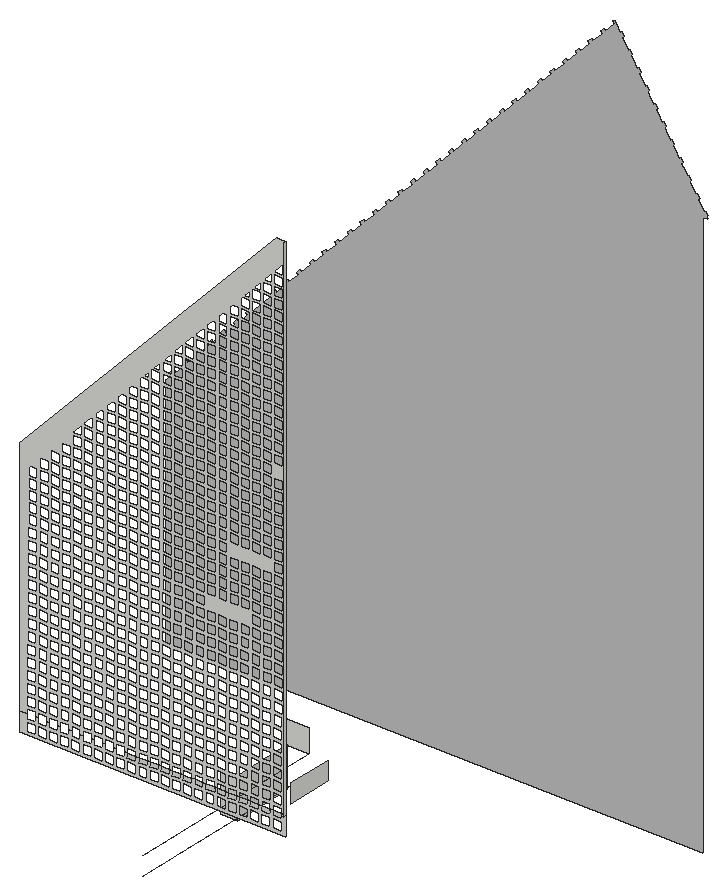
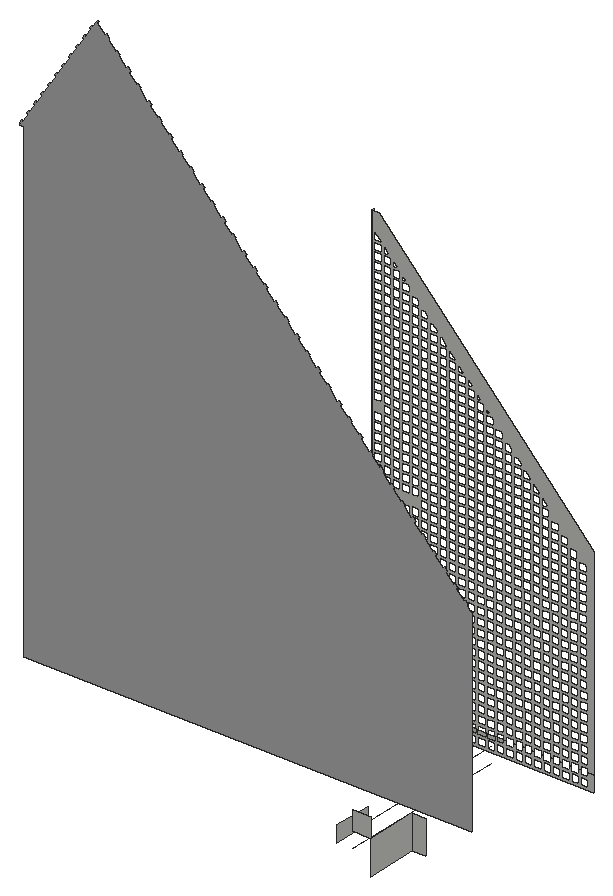
# SketchUp Ruby script. Lengths in inches.
U = 1.inch
M = Sketchup.active_model
def pt(a) = Geom::Point3d.new(a.map { |v| v * U })
def face(e, loops, mat)
  f = e.add_face(loops[0].map { |a| pt(a) })
  loops[1..].each { |l| e.add_face(l.map { |a| pt(a) }).erase! }
  f.material = f.back_material = mat if mat
  f
end
# faces: each face lists its corners as indices into pts; further lists are holes
def faces(e, pts, list, mat = nil) = list.each { |f| face(e, (f[0].is_a?(Array) ? f : [f]).map { |l| l.map { |i| pts[i] } }, mat) }
# xy, xz, yz: faces in a plane at the given z, y or x. An outline is a flat list of corners, or four numbers for a rectangle; further outlines are holes
def ring(l) = l.size == 4 ? [[l[0], l[1]], [l[2], l[1]], [l[2], l[3]], [l[0], l[3]]] : l.each_slice(2).to_a
def flat(e, list, mat, &to3) = list.each { |f| face(e, (f[0].is_a?(Array) ? f : [f]).map { |l| ring(l).map { |u, v| to3.(u, v) } }, mat) }
def xy(e, z, list, mat = nil) = flat(e, list, mat) { |x, y| [x, y, z] }
def xz(e, y, list, mat = nil) = flat(e, list, mat) { |x, z| [x, y, z] }
def yz(e, x, list, mat = nil) = flat(e, list, mat) { |y, z| [x, y, z] }
def lines(e, pts, list) = list.each { |a, b| e.add_line(pt(pts[a]), pt(pts[b])) }
# prism: a flat outline (further loops are holes) pulled along v
def prism(e, loops, v, mat = nil)
  f = face(e, loops, mat); d = Geom::Vector3d.new(v.map { |x| x * U })
  f.pushpull(f.normal.samedirection?(d) ? d.length : -d.length)
end
def box(e, o, s, mat = nil) = prism(e, [[o, [o[0] + s[0], o[1], o[2]], [o[0] + s[0], o[1] + s[1], o[2]], [o[0], o[1] + s[1], o[2]]]], [0, 0, s[2]], mat)
def at(x, y, z, deg = 0) = Geom::Transformation.translation(pt([x, y, z])) * Geom::Transformation.rotation(ORIGIN, Z_AXIS, deg.degrees)
def axes(o, x, y, z) = Geom::Transformation.new([*x, 0, *y, 0, *z, 0, *pt(o).to_a, 1])
def part(name) = M.definitions.add(name)
# library, detail: a bought-in or finely detailed component or shape, given as its bounding box
def library(name, o, s) = part(name).tap { |d| box(d.entities, o, s) }
def detail(e, o, s) = box(e.add_group.entities, o, s)
def put(e, d, t, mat = nil) = e.add_instance(d, t).tap { |i| i.material = mat if mat }
def group(e, t, mat = nil) = e.add_group.tap { |g| g.transformation = t; g.material = mat if mat }.entities
root = M.entities
M.materials.add("[Color M02]").color = [198, 198, 198]
xz(root,480.77,[[[2203.9,258.95,2203.9,263.89,2205.69,263.89,2205.69,262.73,2208,262.73,2208,263.89,2208.6,263.89,2208.6,262.73,2210.92,262.73,2210.92,263.89,2211.52,263.89,2211.52,262.73,2213.83,262.73,2213.83,263.89,2214.43,263.89,2214.43,262.73,2216.74,262.73,2216.74,263.89,2217.34,263.89,2217.34,262.73,2219.65,262.73,2219.65,263.89,2220.25,263.89,2220.25,262.73,2222.5625,262.73,2222.5625,263.89,2223.16,263.89,2223.16,262.73,2225.48,262.73,2225.48,263.89,2226.08,263.89,2226.08,262.73,2228.39,262.73,2228.39,263.89,2228.99,263.89,2228.99,262.73,2231.3,262.73,2231.3,263.89,2231.9,263.89,2231.9,262.73,2234.21,262.73,2234.21,263.89,2234.8125,263.89,2234.8125,262.73,2237.125,262.73,2237.125,263.89,2237.72,263.89,2237.72,262.73,2240.04,262.73,2240.04,263.89,2240.64,263.89,2240.64,262.73,2242.95,262.73,2242.95,263.89,2243.55,263.89,2243.55,262.73,2245.86,262.73,2245.86,263.89,2246.46,263.89,2246.46,262.73,2248.77,262.73,2248.77,263.89,2249.37,263.89,2249.37,262.73,2251.68,262.73,2251.68,263.89,2252.28,263.89,2252.28,262.73,2254.6,262.73,2254.6,263.89,2255.2,263.89,2255.2,262.73,2257.51,262.73,2257.51,263.89,2258.11,263.89,2258.11,262.73,2260.42,262.73,2260.42,263.89,2261.02,263.89,2261.02,262.73,2263.33,262.73,2263.33,263.89,2263.93,263.89,2263.93,262.73,2266.24,262.73,2266.24,263.89,2266.84,263.89,2266.84,262.73,2269.16,262.73,2269.16,263.89,2269.76,263.89,2269.76,262.73,2272.07,262.73,2272.07,263.89,2273.22,263.89,2273.22,258.95],[2269.73,259.68,2272.04,262],[2266.81,259.68,2269.13,262],[2263.9,259.68,2266.22,262],[2260.99,259.68,2263.3,262],[2258.08,259.68,2260.39,262],[2255.17,259.68,2257.48,262],[2252.25,259.68,2254.57,262],[2249.34,259.68,2251.66,262],[2246.43,259.68,2248.74,262],[2243.52,259.68,2245.83,262],[2240.61,259.68,2242.92,262],[2237.69,259.68,2240.01,262],[2234.78,259.68,2237.09,262],[2231.87,259.68,2234.18,262],[2228.96,259.68,2231.27,262],[2226.05,259.68,2228.36,262],[2223.13,259.68,2225.45,262],[2220.22,259.68,2222.53,262],[2217.31,259.68,2219.62,262],[2214.4,259.68,2216.71,262],[2211.49,259.68,2213.8,262],[2208.57,259.68,2210.89,262],[2205.66,259.68,2207.97,262]],[2231.9,262.73,2234.21,263.89],[2234.8125,262.73,2237.125,263.89],[2237.72,262.73,2240.04,263.89],[2240.64,262.73,2242.95,263.89],
  [2243.55,262.73,2245.86,263.89],[2246.46,262.73,2248.77,263.89],[2249.37,262.73,2251.68,263.89],[2252.28,262.73,2254.6,263.89],[2255.2,262.73,2257.51,263.89],
  [2258.11,262.73,2260.42,263.89],[2261.02,262.73,2263.33,263.89],[2263.93,262.73,2266.24,263.89],[2266.84,262.73,2269.16,263.89],[2269.76,262.73,2272.07,263.89],
  [[2203.9,263.89,2203.9,326.5,2270.96,397.75,2273.22,397.75,2273.22,263.89,2272.07,263.89,2272.07,265.04,2269.76,265.04,2269.76,263.89,2269.16,263.89,2269.16,265.04,2266.84,265.04,2266.84,263.89,2266.24,263.89,2266.24,265.04,2263.93,265.04,2263.93,263.89,2263.33,263.89,2263.33,265.04,2261.02,265.04,2261.02,263.89,2260.42,263.89,2260.42,265.04,2258.11,265.04,2258.11,263.89,2257.51,263.89,2257.51,265.04,2255.2,265.04,2255.2,263.89,2254.6,263.89,2254.6,265.04,2252.28,265.04,2252.28,263.89,2251.68,263.89,2251.68,265.04,2249.37,265.04,2249.37,263.89,2248.77,263.89,2248.77,265.04,2246.46,265.04,2246.46,263.89,2245.86,263.89,2245.86,265.04,2243.55,265.04,2243.55,263.89,2242.95,263.89,2242.95,265.04,2240.64,265.04,2240.64,263.89,2240.04,263.89,2240.04,265.04,2237.72,265.04,2237.72,263.89,2237.125,263.89,2237.125,265.04,2234.8125,265.04,2234.8125,263.89,2234.21,263.89,2234.21,265.04,2231.9,265.04,2231.9,263.89,2231.3,263.89,2231.3,265.04,2228.99,265.04,2228.99,263.89,2228.39,263.89,2228.39,265.04,2226.08,265.04,2226.08,263.89,2225.48,263.89,2225.48,265.04,2223.16,265.04,2223.16,263.89,2222.5625,263.89,2222.5625,265.04,2220.25,265.04,2220.25,263.89,2219.65,263.89,2219.65,265.04,2217.34,265.04,2217.34,263.89,2216.74,263.89,2216.74,265.04,2214.43,265.04,2214.43,263.89,2213.83,263.89,2213.83,265.04,2211.52,265.04,2211.52,263.89,2210.92,263.89,2210.92,265.04,2208.6,265.04,2208.6,263.89,2208,263.89,2208,265.04,2205.69,265.04,2205.69,263.89],[2258.52,370.27,2260.86,372.59],[2270.19,386.84,2272.5,389.15],[2270.19,384.09,2272.5,386.4],[2267.28,384.09,2269.59,386.4],[2267.25,381.34,2269.57,383.65],[2270.19,381.34,2272.5,383.65],[2270.19,378.59,2272.5,380.9],[2267.25,378.59,2269.57,380.9],[2264.34,375.84,2266.65,378.15],[2267.28,375.84,2269.59,378.15],[2270.19,375.84,2272.5,378.15],[2270.19,373.09,2272.5,375.4],[2267.25,373.09,2269.57,375.4],[2264.37,373.09,2266.68,375.4],[2261.43,373.09,2263.74,375.4],[2267.25,370.27,2269.57,372.59],[2270.19,370.27,2272.5,372.59],[2261.45,370.27,2263.77,372.59],[2255.63,370.27,2257.94,372.59],[2252.72,367.46,2255.03,369.77],[2255.63,367.46,2257.94,369.77],[2258.54,367.46,2260.86,369.77],[2261.45,367.46,2263.77,369.77],[2264.37,367.46,2266.68,369.77],[2267.28,367.46,2269.59,369.77],[2270.19,367.46,2272.5,369.77],[2270.19,364.65,2272.5,366.96],[2267.28,364.65,2269.59,366.96],[2264.37,364.65,2266.68,366.96],[2261.45,364.65,2263.77,366.96],[2258.54,364.65,2260.86,366.96],[2255.63,364.65,2257.94,366.96],[2252.72,364.65,2255.03,366.96],[2249.81,364.65,2252.12,366.96],[2246.89,361.84,2249.21,364.15],[2249.81,361.84,2252.12,364.15],[2252.72,361.84,2255.03,364.15],[2255.63,361.84,2257.94,364.15],[2258.54,361.84,2260.86,364.15],[2261.45,361.84,2263.77,364.15],[2264.37,361.84,2266.68,364.15],[2267.28,361.84,2269.59,364.15],[2270.19,361.84,2272.5,364.15],[2270.19,359.02,2272.5,361.34],[2267.28,359.02,2269.59,361.34],[2264.37,359.02,2266.68,361.34],[2261.45,359.02,2263.77,361.34],[2258.54,359.02,2260.86,361.34],[2255.63,359.02,2257.94,361.34],[2252.72,359.02,2255.03,361.34],[2249.81,359.02,2252.12,361.34],[2246.89,359.02,2249.21,361.34],[2243.98,359.02,2246.29,361.34],[2241.07,356.21,2243.38,358.52],[2243.98,356.21,2246.29,358.52],[2246.89,356.21,2249.21,358.52],[2249.81,356.21,2252.12,358.52],[2252.72,356.21,2255.03,358.52],[2255.63,356.21,2257.94,358.52],[2258.54,356.21,2260.86,358.52],[2261.45,356.21,2263.77,358.52],[2264.37,356.21,2266.68,358.52],[2267.28,356.21,2269.59,358.52],[2270.19,356.21,2272.5,358.52],[2238.16,350.59,2240.47,352.9],[2241.07,353.4,2243.38,355.71],[2241.07,350.59,2243.38,352.9],[2243.98,350.59,2246.29,352.9],[2243.98,353.4,2246.29,355.71],[2246.89,353.4,2249.21,355.71],[2246.89,350.59,2249.21,352.9],[2249.81,353.4,2252.12,355.71],[2249.81,350.59,2252.12,352.9],[2252.72,353.4,2255.03,355.71],[2252.72,350.59,2255.03,352.9],[2255.63,353.4,2257.94,355.71],[2255.63,350.59,2257.94,352.9],[2258.54,353.4,2260.86,355.71],[2258.54,350.59,2260.86,352.9],[2261.45,350.59,2263.77,352.9],[2261.45,353.4,2263.77,355.71],[2264.37,353.4,2266.68,355.71],[2267.28,353.4,2269.59,355.71],[2270.19,353.4,2272.5,355.71],[2270.19,350.59,2272.5,352.9],[2267.28,350.59,2269.59,352.9],[2264.37,350.59,2266.68,352.9],[2270.19,347.77,2272.5,350.09],[2267.28,347.77,2269.59,350.09],[2264.37,347.77,2266.68,350.09],[2261.45,347.77,2263.77,350.09],[2258.54,347.77,2260.86,350.09],[2255.63,347.77,2257.94,350.09],[2252.72,347.77,2255.03,350.09],[2249.81,347.77,2252.12,350.09],[2246.89,347.77,2249.21,350.09],[2243.98,347.77,2246.29,350.09],[2241.07,347.77,2243.38,350.09],[2238.16,347.77,2240.47,350.09],[2235.25,347.77,2237.56,350.09],[2232.33,344.96,2234.65,347.27],[2235.25,344.96,2237.56,347.27],[2238.16,344.96,2240.47,347.27],[2241.07,344.96,2243.38,347.27],[2243.98,344.96,2246.29,347.27],[2246.89,344.96,2249.21,347.27],[2249.81,344.96,2252.12,347.27],[2252.72,344.96,2255.03,347.27],[2255.63,344.96,2257.94,347.27],[2258.54,344.96,2260.86,347.27],[2261.45,344.96,2263.77,347.27],[2264.37,344.96,2266.68,347.27],[2267.28,344.96,2269.59,347.27],[2270.19,344.96,2272.5,347.27],[2223.6,336.52,2225.91,338.84],[2226.51,336.52,2228.82,338.84],[2229.42,336.52,2231.73,338.84],[2232.33,336.52,2234.65,338.84],[2235.25,336.52,2237.56,338.84],[2238.16,336.52,2240.47,338.84],[2241.07,336.52,2243.38,338.84],[2243.98,336.52,2246.29,338.84],[2246.89,336.52,2249.21,338.84],[2249.81,336.52,2252.12,338.84],[2249.81,339.34,2252.12,341.65],[2246.89,339.34,2249.21,341.65],[2243.98,339.34,2246.29,341.65],[2241.07,339.34,2243.38,341.65],[2238.16,339.34,2240.47,341.65],[2235.25,339.34,2237.56,341.65],[2232.33,339.34,2234.65,341.65],[2229.42,339.34,2231.73,341.65],[2226.51,339.34,2228.82,341.65],[2229.42,342.15,2231.73,344.46],[2232.33,342.15,2234.65,344.46],[2235.25,342.15,2237.56,344.46],[2238.16,342.15,2240.47,344.46],[2241.07,342.15,2243.38,344.46],[2243.98,342.15,2246.29,344.46],[2246.89,342.15,2249.21,344.46],[2249.81,342.15,2252.12,344.46],[2252.72,342.15,2255.03,344.46],[2252.72,339.34,2255.03,341.65],[2252.72,336.52,2255.03,338.84],[2255.63,336.52,2257.94,338.84],[2255.63,339.34,2257.94,341.65],[2255.63,342.15,2257.94,344.46],[2258.54,342.15,2260.86,344.46],[2258.54,339.34,2260.86,341.65],[2258.54,336.52,2260.86,338.84],[2261.45,336.52,2263.77,338.84],[2261.45,339.34,2263.77,341.65],[2261.45,342.15,2263.77,344.46],[2264.37,342.15,2266.68,344.46],[2264.37,339.34,2266.68,341.65],[2264.37,336.52,2266.68,338.84],[2267.28,336.52,2269.59,338.84],[2267.28,339.34,2269.59,341.65],[2267.28,342.15,2269.59,344.46],[2270.19,339.34,2272.5,341.65],[2270.19,336.52,2272.5,338.84],[2270.19,333.71,2272.5,336.02],[2267.28,333.71,2269.59,336.02],[2264.37,333.71,2266.68,336.02],[2261.45,333.71,2263.77,336.02],[2258.54,333.71,2260.86,336.02],[2255.63,333.71,2257.94,336.02],[2252.72,333.71,2255.03,336.02],[2249.81,333.71,2252.12,336.02],[2246.89,333.71,2249.21,336.02],[2243.98,333.71,2246.29,336.02],[2241.07,333.71,2243.38,336.02],[2238.16,333.71,2240.47,336.02],[2235.25,333.71,2237.56,336.02],[2232.33,333.71,2234.65,336.02],[2229.42,333.71,2231.73,336.02],[2226.51,333.71,2228.82,336.02],[2223.6,333.71,2225.91,336.02],[2220.6875,333.71,2223,336.02],[2217.77,330.9,2220.09,333.21],[2220.6875,330.9,2223,333.21],[2223.6,330.9,2225.91,333.21],[2226.51,330.9,2228.82,333.21],[2229.42,330.9,2231.73,333.21],[2232.33,330.9,2234.65,333.21],[2235.25,330.9,2237.56,333.21],[2238.16,330.9,2240.47,333.21],[2241.07,330.9,2243.38,333.21],[2243.98,330.9,2246.29,333.21],[2246.89,330.9,2249.21,333.21],[2249.81,330.9,2252.12,333.21],[2252.72,330.9,2255.03,333.21],[2255.63,330.9,2257.94,333.21],[2258.54,330.9,2260.86,333.21],[2261.45,330.9,2263.77,333.21],[2264.37,330.9,2266.68,333.21],[2267.28,330.9,2269.59,333.21],[2270.19,330.9,2272.5,333.21],[2270.19,328.09,2272.5,330.4],[2267.28,328.09,2269.59,330.4],[2264.37,328.09,2266.68,330.4],[2261.45,328.09,2263.77,330.4],[2258.54,328.09,2260.86,330.4],[2255.63,328.09,2257.94,330.4],[2252.72,328.09,2255.03,330.4],[2249.81,328.09,2252.12,330.4],[2246.89,328.09,2249.21,330.4],[2243.98,328.09,2246.29,330.4],[2241.07,328.09,2243.38,330.4],[2238.16,328.09,2240.47,330.4],[2235.25,328.09,2237.56,330.4],[2232.33,328.09,2234.65,330.4],[2229.42,328.09,2231.73,330.4],[2226.51,328.09,2228.82,330.4],[2223.6,328.09,2225.91,330.4],[2220.6875,328.09,2223,330.4],[2217.77,328.09,2220.09,330.4],[2214.86,328.09,2217.17,330.4],[2211.95,325.27,2214.26,327.59],[2214.86,325.27,2217.17,327.59],[2217.77,325.27,2220.09,327.59],[2220.6875,325.27,2223,327.59],[2223.6,325.27,2225.91,327.59],[2226.51,325.27,2228.82,327.59],[2229.42,325.27,2231.73,327.59],[2232.33,325.27,2234.65,327.59],[2235.25,325.27,2237.56,327.59],[2238.16,325.27,2240.47,327.59],[2241.07,325.27,2243.38,327.59],[2243.98,325.27,2246.29,327.59],[2246.89,325.27,2249.21,327.59],[2249.81,325.27,2252.12,327.59],[2252.72,325.27,2255.03,327.59],[2255.63,325.27,2257.94,327.59],[2258.54,325.27,2260.86,327.59],[2261.45,325.27,2263.77,327.59],[2264.37,325.27,2266.68,327.59],[2267.28,325.27,2269.59,327.59],[2270.19,325.27,2272.5,327.59],[2270.19,322.46,2272.5,324.77],[2267.28,322.46,2269.59,324.77],[2264.37,322.46,2266.68,324.77],[2261.45,322.46,2263.77,324.77],[2258.54,322.46,2260.86,324.77],[2255.63,322.46,2257.94,324.77],[2252.72,322.46,2255.03,324.77],[2249.81,322.46,2252.12,324.77],[2246.89,322.46,2249.21,324.77],[2243.98,322.46,2246.29,324.77],[2241.07,322.46,2243.38,324.77],[2238.16,322.46,2240.47,324.77],[2235.25,322.46,2237.56,324.77],[2232.33,322.46,2234.65,324.77],[2232.33,319.65,2234.65,321.96],[2235.25,319.65,2237.56,321.96],[2238.16,319.65,2240.47,321.96],[2241.07,319.65,2243.38,321.96],[2243.98,319.65,2246.29,321.96],[2246.89,319.65,2249.21,321.96],[2249.81,319.65,2252.12,321.96],[2252.72,319.65,2255.03,321.96],[2255.63,319.65,2257.94,321.96],[2270.19,319.65,2272.5,321.96],[2270.19,316.84,2272.5,319.15],[2267.28,316.84,2269.59,319.15],[2264.37,316.84,2266.68,319.15],[2261.45,316.84,2263.77,319.15],[2258.54,316.84,2260.86,319.15],[2255.63,316.84,2257.94,319.15],[2252.72,316.84,2255.03,319.15],[2249.81,316.84,2252.12,319.15],[2246.89,316.84,2249.21,319.15],[2243.98,316.84,2246.29,319.15],[2241.07,316.84,2243.38,319.15],[2238.16,316.84,2240.47,319.15],[2235.25,316.84,2237.56,319.15],[2232.33,316.84,2234.65,319.15],[2232.33,314.02,2234.65,316.34],[2235.25,314.02,2237.56,316.34],[2238.16,314.02,2240.47,316.34],[2241.07,314.02,2243.38,316.34],[2243.98,314.02,2246.29,316.34],[2246.89,314.02,2249.21,316.34],[2249.81,314.02,2252.12,316.34],[2252.72,314.02,2255.03,316.34],[2255.63,314.02,2257.94,316.34],[2258.54,314.02,2260.86,316.34],[2261.45,314.02,2263.77,316.34],[2264.37,314.02,2266.68,316.34],[2267.28,314.02,2269.59,316.34],[2270.19,314.02,2272.5,316.34],[2211.95,322.46,2214.26,324.77],[2214.86,322.46,2217.17,324.77],[2217.77,322.46,2220.09,324.77],[2220.6875,322.46,2223,324.77],[2223.6,322.46,2225.91,324.77],[2226.51,322.46,2228.82,324.77],[2229.42,322.46,2231.73,324.77],[2229.42,319.65,2231.73,321.96],[2229.42,316.84,2231.73,319.15],[2229.42,314.02,2231.73,316.34],[2226.51,314.02,2228.82,316.34],[2226.51,316.84,2228.82,319.15],[2226.51,319.65,2228.82,321.96],[2223.6,319.65,2225.91,321.96],[2220.6875,319.65,2223,321.96],[2217.77,319.65,2220.09,321.96],[2214.86,319.65,2217.17,321.96],[2211.95,319.65,2214.26,321.96],[2209.04,319.65,2211.35,321.96],[2206.125,316.84,2208.4375,319.15],[2209.04,316.84,2211.35,319.15],[2211.95,316.84,2214.26,319.15],[2214.86,316.84,2217.17,319.15],[2217.77,316.84,2220.09,319.15],[2220.6875,316.84,2223,319.15],[2223.6,316.84,2225.91,319.15],[2223.6,314.02,2225.91,316.34],[2220.6875,314.02,2223,316.34],[2217.77,314.02,2220.09,316.34],[2214.86,314.02,2217.17,316.34],[2211.95,314.02,2214.26,316.34],[2209.04,314.02,2211.35,316.34],[2206.125,314.02,2208.4375,316.34],[2206.125,311.21,2208.4375,313.52],[2209.04,311.21,2211.35,313.52],[2211.95,311.21,2214.26,313.52],[2214.86,311.21,2217.17,313.52],[2217.77,311.21,2220.09,313.52],[2220.6875,311.21,2223,313.52],[2223.6,311.21,2225.91,313.52],[2226.51,311.21,2228.82,313.52],[2229.42,311.21,2231.73,313.52],[2232.33,311.21,2234.65,313.52],[2235.25,311.21,2237.56,313.52],[2238.16,311.21,2240.47,313.52],[2241.07,311.21,2243.38,313.52],[2243.98,311.21,2246.29,313.52],[2246.89,311.21,2249.21,313.52],[2249.81,311.21,2252.12,313.52],[2252.72,311.21,2255.03,313.52],[2255.63,311.21,2257.94,313.52],[2258.54,311.21,2260.86,313.52],[2261.45,311.21,2263.77,313.52],[2264.37,311.21,2266.68,313.52],[2267.28,311.21,2269.59,313.52],[2270.19,311.21,2272.5,313.52],[2206.125,308.4,2208.4375,310.71],[2209.04,308.4,2211.35,310.71],[2211.95,308.4,2214.26,310.71],[2214.86,308.4,2217.17,310.71],[2217.77,308.4,2220.09,310.71],[2220.6875,308.4,2223,310.71],[2223.6,308.4,2225.91,310.71],[2226.51,308.4,2228.82,310.71],[2229.42,308.4,2231.73,310.71],[2232.33,308.4,2234.65,310.71],[2235.25,308.4,2237.56,310.71],[2238.16,308.4,2240.47,310.71],[2241.07,308.4,2243.38,310.71],[2243.98,308.4,2246.29,310.71],[2246.89,308.4,2249.21,310.71],[2249.81,308.4,2252.12,310.71],[2252.72,308.4,2255.03,310.71],[2255.63,308.4,2257.94,310.71],[2258.54,308.4,2260.86,310.71],[2261.45,308.4,2263.77,310.71],[2264.37,308.4,2266.68,310.71],[2267.28,308.4,2269.59,310.71],[2270.19,308.4,2272.5,310.71],[2270.16,305.35,2272.47,307.67],[2267.25,305.35,2269.5625,307.67],[2264.34,305.35,2266.65,307.67],[2249.78,305.35,2252.09,307.67],[2246.87,305.35,2249.18,307.67],[2243.95,305.35,2246.27,307.67],[2241.04,305.35,2243.35,307.67],[2238.13,305.35,2240.44,307.67],[2235.22,305.35,2237.53,307.67],[2232.31,305.35,2234.62,307.67],[2229.39,305.35,2231.71,307.67],[2226.48,305.35,2228.79,307.67],[2223.57,305.35,2225.88,307.67],[2220.66,305.35,2222.97,307.67],[2217.75,305.35,2220.06,307.67],[2214.83,305.35,2217.15,307.67],[2211.92,305.35,2214.23,307.67],[2209.01,305.35,2211.32,307.67],[2206.1,305.35,2208.41,307.67],[2206.07,302.31,2208.38,304.62],[2208.98,302.31,2211.29,304.62],[2211.89,302.31,2214.2,304.62],[2214.8,302.31,2217.12,304.62],[2217.72,302.31,2220.03,304.62],[2220.63,302.31,2222.94,304.62],[2223.54,302.31,2225.85,304.62],[2226.45,302.31,2228.76,304.62],[2229.36,302.31,2231.68,304.62],[2232.28,302.31,2234.59,304.62],[2235.1875,302.31,2237.5,304.62],[2238.1,302.31,2240.41,304.62],[2241.01,302.31,2243.32,304.62],[2243.92,302.31,2246.24,304.62],[2246.84,302.31,2249.15,304.62],[2249.75,302.31,2252.0625,304.62],[2252.66,302.31,2254.97,304.62],[2255.57,302.31,2257.89,304.62],[2258.48,302.31,2260.8,304.62],[2261.4,302.31,2263.71,304.62],[2264.31,302.31,2266.62,304.62],[2267.22,302.31,2269.53,304.62],[2270.13,302.31,2272.45,304.62],[2270.1,299.27,2272.42,301.58],[2267.19,299.27,2269.5,301.58],[2264.28,299.27,2266.59,301.58],[2261.37,299.27,2263.68,301.58],[2258.46,299.27,2260.77,301.58],[2255.54,299.27,2257.86,301.58],[2252.63,299.27,2254.94,301.58],[2249.72,299.27,2252.03,301.58],[2246.81,299.27,2249.12,301.58],[2243.9,299.27,2246.21,301.58],[2240.98,299.27,2243.3,301.58],[2238.07,299.27,2240.38,301.58],[2235.16,299.27,2237.47,301.58],[2232.25,299.27,2234.56,301.58],[2229.34,299.27,2231.65,301.58],[2226.42,299.27,2228.74,301.58],[2223.51,299.27,2225.82,301.58],[2220.6,299.27,2222.91,301.58],[2217.6875,299.27,2220,301.58],[2214.78,299.27,2217.09,301.58],[2211.86,299.27,2214.18,301.58],[2208.95,299.27,2211.26,301.58],[2206.04,299.27,2208.35,301.58],[2206.01,296.22,2208.32,298.53],[2208.92,296.22,2211.23,298.53],[2211.83,296.22,2214.15,298.53],[2214.75,296.22,2217.06,298.53],[2217.66,296.22,2219.97,298.53],[2220.57,296.22,2222.88,298.53],[2223.48,296.22,2225.79,298.53],[2226.39,296.22,2228.71,298.53],[2229.31,296.22,2231.62,298.53],[2232.22,296.22,2234.53,298.53],[2235.13,296.22,2237.44,298.53],[2238.04,296.22,2240.35,298.53],[2240.95,296.22,2243.27,298.53],[2243.87,296.22,2246.18,298.53],[2246.78,296.22,2249.09,298.53],[2249.69,296.22,2252,298.53],[2252.6,296.22,2254.91,298.53],[2255.51,296.22,2257.83,298.53],[2258.43,296.22,2260.74,298.53],[2261.34,296.22,2263.65,298.53],[2264.25,296.22,2266.5625,298.53],[2267.16,296.22,2269.48,298.53],[2270.07,296.22,2272.39,298.53],[2205.98,293.18,2208.29,295.49],[2208.89,293.18,2211.21,295.49],[2211.8,293.18,2214.12,295.49],[2214.72,293.18,2217.03,295.49],[2217.63,293.18,2219.94,295.49],[2220.54,293.18,2222.85,295.49],[2223.45,293.18,2225.77,295.49],[2226.37,293.18,2228.68,295.49],[2229.28,293.18,2231.59,295.49],[2232.1875,293.18,2234.5,295.49],[2235.1,293.18,2237.41,295.49],[2238.01,293.18,2240.33,295.49],[2240.93,293.18,2243.24,295.49],[2243.84,293.18,2246.15,295.49],[2246.75,293.18,2249.0625,295.49],[2249.66,293.18,2251.97,295.49],[2252.57,293.18,2254.89,295.49],[2255.49,293.18,2257.8,295.49],[2258.4,293.18,2260.71,295.49],[2261.31,293.18,2263.62,295.49],[2264.22,293.18,2266.53,295.49],[2267.13,293.18,2269.45,295.49],[2270.05,293.18,2272.36,295.49],[2217.6,290.13,2219.91,292.44],[2220.51,290.13,2222.82,292.44],[2223.42,290.13,2225.74,292.44],[2226.34,290.13,2228.65,292.44],[2229.25,290.13,2231.5625,292.44],[2232.16,290.13,2234.47,292.44],[2235.07,290.13,2237.38,292.44],[2237.98,290.13,2240.3,292.44],[2240.9,290.13,2243.21,292.44],[2243.81,290.13,2246.12,292.44],[2246.72,290.13,2249.03,292.44],[2249.63,290.13,2251.94,292.44],[2252.54,290.13,2254.86,292.44],[2255.46,290.13,2257.77,292.44],[2258.37,290.13,2260.68,292.44],[2261.28,290.13,2263.59,292.44],[2264.19,290.13,2266.51,292.44],[2267.1,290.13,2269.42,292.44],[2270.02,290.13,2272.33,292.44],[2269.99,287.09,2272.3,289.4],[2267.08,287.09,2269.39,289.4],[2264.16,287.09,2266.48,289.4],[2261.25,287.09,2263.5625,289.4],[2258.34,287.09,2260.65,289.4],[2255.43,287.09,2257.74,289.4],[2252.52,287.09,2254.83,289.4],[2249.6,287.09,2251.92,289.4],[2246.69,287.09,2249,289.4],[2243.78,287.09,2246.09,289.4],[2240.87,287.09,2243.18,289.4],[2237.96,287.09,2240.27,289.4],[2235.04,287.09,2237.36,289.4],[2232.13,287.09,2234.44,289.4],[2229.22,287.09,2231.53,289.4],[2226.31,287.09,2228.62,289.4],[2223.4,287.09,2225.71,289.4],[2220.48,287.09,2222.8,289.4],[2217.57,287.09,2219.88,289.4],[2217.54,284.04,2219.85,286.35],[2220.45,284.04,2222.77,286.35],[2223.37,284.04,2225.68,286.35],[2226.28,284.04,2228.59,286.35],[2229.19,284.04,2231.5,286.35],[2232.1,284.04,2234.41,286.35],[2235.01,284.04,2237.33,286.35],[2237.93,284.04,2240.24,286.35],[2240.84,284.04,2243.15,286.35],[2243.75,284.04,2246.0625,286.35],[2246.66,284.04,2248.97,286.35],[2249.57,284.04,2251.89,286.35],[2252.49,284.04,2254.8,286.35],[2255.4,284.04,2257.71,286.35],[2258.3125,284.04,2260.625,286.35],[2261.22,284.04,2263.54,286.35],[2264.13,284.04,2266.45,286.35],[2267.05,284.04,2269.36,286.35],[2269.96,284.04,2272.27,286.35],[2269.93,281,2272.24,283.31],[2267.02,281,2269.33,283.31],[2264.11,281,2266.42,283.31],[2261.19,281,2263.51,283.31],[2258.28,281,2260.59,283.31],[2255.37,281,2257.68,283.31],[2252.46,281,2254.77,283.31],[2249.55,281,2251.86,283.31],[2246.63,281,2248.95,283.31],[2243.72,281,2246.03,283.31],[2240.81,281,2243.12,283.31],[2237.9,281,2240.21,283.31],[2234.99,281,2237.3,283.31],[2232.07,281,2234.39,283.31],[2229.16,281,2231.47,283.31],[2226.25,281,2228.5625,283.31],[2223.34,281,2225.65,283.31],[2220.43,281,2222.74,283.31],[2220.4,277.95,2222.71,280.26],[2223.31,277.95,2225.62,280.26],[2226.22,277.95,2228.53,280.26],[2229.13,277.95,2231.44,280.26],[2232.04,277.95,2234.36,280.26],[2234.96,277.95,2237.27,280.26],[2237.87,277.95,2240.18,280.26],[2240.78,277.95,2243.09,280.26],[2243.69,277.95,2246,280.26],[2246.6,277.95,2248.92,280.26],[2249.52,277.95,2251.83,280.26],[2252.43,277.95,2254.74,280.26],[2255.34,277.95,2257.65,280.26],[2258.25,277.95,2260.57,280.26],[2261.16,277.95,2263.48,280.26],[2264.08,277.95,2266.39,280.26],[2266.99,277.95,2269.3,280.26],[2269.9,277.95,2272.21,280.26],[2269.87,274.91,2272.18,277.22],[2266.96,274.91,2269.27,277.22],[2264.05,274.91,2266.36,277.22],[2261.14,274.91,2263.45,277.22],[2258.22,274.91,2260.54,277.22],[2255.3125,274.91,2257.625,277.22],[2252.4,274.91,2254.71,277.22],[2249.49,274.91,2251.8,277.22],[2246.58,274.91,2248.89,277.22],[2243.66,274.91,2245.98,277.22],[2240.75,274.91,2243.0625,277.22],[2237.84,274.91,2240.15,277.22],[2234.93,274.91,2237.24,277.22],[2232.02,274.91,2234.33,277.22],[2229.1,274.91,2231.42,277.22],[2226.19,274.91,2228.5,277.22],[2223.28,274.91,2225.59,277.22],[2220.37,274.91,2222.68,277.22],[2217.51,281,2219.83,283.31],[2217.48,277.95,2219.8,280.26],[2217.46,274.91,2219.77,277.22],[2214.54,274.91,2216.86,277.22],[2214.57,277.95,2216.88,280.26],[2214.6,281,2216.91,283.31],[2214.63,284.04,2216.94,286.35],[2214.66,287.09,2216.97,289.4],[2214.6875,290.13,2217,292.44],[2211.78,290.13,2214.09,292.44],[2211.75,287.09,2214.06,289.4],[2211.72,284.04,2214.03,286.35],[2211.6875,281,2214,283.31],[2208.75,277.95,2211.06,280.26],[2211.66,277.95,2213.97,280.26],[2211.63,274.91,2213.94,277.22],[2208.72,274.91,2211.03,277.22],[2208.78,281,2211.09,283.31],[2208.81,284.04,2211.12,286.35],[2208.83,287.09,2211.15,289.4],[2208.86,290.13,2211.18,292.44],[2205.95,290.13,2208.26,292.44],[2205.92,287.09,2208.24,289.4],[2205.89,284.04,2208.21,286.35],[2205.86,281,2208.18,283.31],[2205.84,277.95,2208.15,280.26],[2205.81,274.91,2208.12,277.22],[2205.78,271.86,2208.09,274.17],[2208.69,271.86,2211,274.17],[2211.6,271.86,2213.91,274.17],[2214.51,271.86,2216.83,274.17],[2217.43,271.86,2219.74,274.17],[2220.34,271.86,2222.65,274.17],[2223.25,271.86,2225.5625,274.17],[2226.16,271.86,2228.47,274.17],[2229.07,271.86,2231.39,274.17],[2231.99,271.86,2234.3,274.17],[2234.9,271.86,2237.21,274.17],[2237.81,271.86,2240.12,274.17],[2240.72,271.86,2243.03,274.17],[2243.63,271.86,2245.95,274.17],[2246.55,271.86,2248.86,274.17],[2249.46,271.86,2251.77,274.17],[2252.37,271.86,2254.68,274.17],[2255.28,271.86,2257.6,274.17],[2258.19,271.86,2260.51,274.17],[2261.11,271.86,2263.42,274.17],[2264.02,271.86,2266.33,274.17],[2266.93,271.86,2269.24,274.17],[2269.84,271.86,2272.16,274.17],[2269.8125,268.82,2272.125,271.13],[2266.9,268.82,2269.21,271.13],[2263.99,268.82,2266.3,271.13],[2261.08,268.82,2263.39,271.13],[2258.17,268.82,2260.48,271.13],[2255.25,268.82,2257.57,271.13],[2252.34,268.82,2254.65,271.13],[2249.43,268.82,2251.74,271.13],[2246.52,268.82,2248.83,271.13],[2243.61,268.82,2245.92,271.13],[2240.69,268.82,2243.01,271.13],[2237.78,268.82,2240.09,271.13],[2234.87,268.82,2237.18,271.13],[2231.96,268.82,2234.27,271.13],[2229.05,268.82,2231.36,271.13],[2226.13,268.82,2228.45,271.13],[2223.22,268.82,2225.53,271.13],[2220.31,268.82,2222.62,271.13],[2217.4,268.82,2219.71,271.13],[2214.49,268.82,2216.8,271.13],[2211.57,268.82,2213.89,271.13],[2208.66,268.82,2210.97,271.13],[2205.75,268.82,2208.0625,271.13],[2205.72,265.77,2208.03,268.09],[2208.63,265.77,2210.94,268.09],[2211.54,265.77,2213.86,268.09],[2214.46,265.77,2216.77,268.09],[2217.37,265.77,2219.68,268.09],[2220.28,265.77,2222.59,268.09],[2223.19,265.77,2225.5,268.09],[2226.1,265.77,2228.42,268.09],[2229.02,265.77,2231.33,268.09],[2231.93,265.77,2234.24,268.09],[2234.84,265.77,2237.15,268.09],[2237.75,265.77,2240.06,268.09],[2240.66,265.77,2242.98,268.09],[2243.58,265.77,2245.89,268.09],[2246.49,265.77,2248.8,268.09],[2249.4,265.77,2251.71,268.09],[2252.3125,265.77,2254.625,268.09],[2255.22,265.77,2257.54,268.09],[2258.14,265.77,2260.45,268.09],[2261.05,265.77,2263.36,268.09],[2263.96,265.77,2266.27,268.09],[2266.87,265.77,2269.19,268.09],[2269.78,265.77,2272.1,268.09],[2264.37,381.34,2266.68,381.34,2266.68,383.65,2264.48,383.65,2264.37,383.53],[2264.37,378.59,2266.68,378.59,2266.68,380.9,2264.48,380.9,2264.37,380.78],[2261.45,375.84,2263.77,375.84,2263.77,378.15,2261.5625,378.15,2261.45,378.03],[2258.54,373.09,2260.86,373.09,2260.86,375.4,2258.65,375.4,2258.54,375.28],[2264.37,370.27,2266.68,370.27,2266.68,372.59,2264.48,372.59,2264.37,372.47],[2238.16,353.4,2240.47,353.4,2240.47,355.71,2238.29,355.71,2238.16,355.57],[2209.04,322.46,2211.35,322.46,2211.35,324.77,2209.29,324.77,2209.04,324.5],[2235.25,350.59,2237.56,350.59,2237.56,352.9,2235.65,352.9,2235.25,352.46],[2261.45,378.59,2263.77,378.59,2263.77,380.9,2261.9,380.9,2261.45,380.43],[2206.125,319.65,2208.4375,319.65,2208.4375,321.96,2206.66,321.96,2206.125,321.39],[2232.33,347.77,2234.65,347.77,2234.65,350.09,2233.02,350.09,2232.33,349.36],[2258.54,375.84,2260.86,375.84,2260.86,378.15,2259.32,378.15,2258.54,377.32],[2229.42,344.96,2231.73,344.96,2231.73,347.27,2230.38,347.27,2229.42,346.25],[2255.63,373.09,2257.94,373.09,2257.94,375.4,2256.74,375.4,2255.63,374.21],[2226.51,342.15,2228.82,342.15,2228.82,344.46,2227.75,344.46,2226.51,343.14],[2252.72,370.27,2255.03,370.27,2255.03,372.59,2254.11,372.59,2252.72,371.11],[2223.6,339.34,2225.91,339.34,2225.91,341.65,2225.11,341.65,2223.6,340.04],[2249.81,367.46,2252.12,367.46,2252.12,369.77,2251.47,369.77,2249.81,368],[2220.6875,336.52,2223,336.52,2223,338.84,2222.47,338.84,2220.6875,336.93],[2246.89,364.65,2249.21,364.65,2249.21,366.96,2248.83,366.96,2246.89,364.89],[2270.19,389.59,2272.5,389.59,2272.5,391.9,2272.21,391.9,2270.19,389.75],[2217.77,333.71,2220.09,333.71,2220.09,336.02,2219.84,336.02,2217.77,333.82],[2244.03,361.84,2246.29,361.84,2246.29,364.15,2246.2,364.15],[2267.46,386.84,2269.59,386.84,2269.59,389.11],[2241.4,359.02,2243.38,359.02,2243.38,361.14],[2264.89,384.09,2266.68,384.09,2266.68,386],[2238.76,356.21,2240.47,356.21,2240.47,358.04],[2262.31,381.34,2263.77,381.34,2263.77,382.89],[2236.12,353.4,2237.56,353.4,2237.56,354.93]]])
xz(root,505.3125,[[2236.57,240.47,2240.94,251.0625]])
xz(root,521.5625,[[2240.94,251.0625,2246.66,257.0625]])
xz(root,521.5625,[[2209.43,263.89,2349.23,263.89,2349.23,412.22,2350.46,412.22,2350.16,412.6875,2350.53,412.92,2349.98,413.79,2349.61,413.55,2348.42,415.41,2347.97,416.11,2348.34,416.34,2347.79,417.21,2347.42,416.97,2346.23,418.83,2345.78,419.53,2346.15,419.76,2345.59,420.63,2345.22,420.39,2344.04,422.25,2343.59,422.95,2343.96,423.18,2343.4,424.05,2343.03,423.8125,2341.84,425.67,2341.39,426.37,2341.76,426.6,2341.21,427.47,2340.84,427.23,2339.65,429.09,2339.2,429.79,2339.57,430.02,2339.02,430.89,2338.65,430.65,2337.46,432.51,2337.01,433.21,2337.38,433.44,2336.82,434.31,2336.45,434.07,2335.27,435.93,2334.82,436.63,2335.18,436.86,2334.63,437.73,2334.26,437.49,2333.07,439.35,2332.625,440.05,2332.99,440.28,2332.4375,441.15,2332.07,440.91,2330.88,442.77,2330.43,443.47,2330.8,443.7,2330.24,444.57,2329.875,444.33,2328.6875,446.1875,2328.24,446.89,2328.61,447.125,2328.05,447.99,2327.68,447.75,2326.5,449.61,2326.17,450.11,2325.9,449.82,2326.36,449.39,2323.9375,446.82,2323.48,447.25,2322.61,446.32,2323.0625,445.89,2320.64,443.32,2320.19,443.75,2319.31,442.8125,2319.76,442.39,2317.34,439.8125,2316.89,440.24,2316.01,439.31,2316.46,438.88,2314.04,436.31,2313.59,436.74,2312.71,435.81,2313.17,435.38,2310.74,432.81,2310.29,433.23,2309.41,432.3,2309.87,431.875,2307.45,429.3,2306.99,429.73,2306.11,428.8,2306.57,428.37,2304.15,425.8,2303.69,426.23,2302.81,425.29,2303.27,424.86,2300.85,422.29,2300.39,422.72,2299.52,421.79,2299.97,421.36,2297.55,418.79,2297.1,419.22,2296.22,418.28,2296.67,417.86,2294.25,415.28,2293.8,415.71,2292.92,414.78,2293.375,414.35,2290.95,411.78,2290.5,412.21,2289.62,411.28,2290.08,410.85,2287.65,408.28,2287.2,408.7,2286.32,407.77,2286.78,407.34,2284.36,404.77,2283.9,405.2,2283.02,404.27,2283.48,403.84,2281.06,401.27,2280.6,401.7,2279.73,400.76,2280.18,400.34,2277.76,397.76,2277.3,398.19,2276.43,397.26,2276.88,396.83,2274.46,394.26,2274.01,394.6875,2273.13,393.75,2273.58,393.33,2271.16,390.75,2270.71,391.18,2269.83,390.25,2270.28,389.82,2267.86,387.25,2267.41,387.68,2266.53,386.75,2266.99,386.32,2264.56,383.75,2264.11,384.17,2263.23,383.24,2263.6875,382.8125,2261.27,380.24,2260.8125,380.67,2259.93,379.74,2260.39,379.31,2257.97,376.74,2257.51,377.17,2256.64,376.23,2257.09,375.81,2254.67,373.23,2254.21,373.66,2253.34,372.73,2253.79,372.3,2251.37,369.73,2250.92,370.16,2250.04,369.23,2250.49,368.8,2248.07,366.22,2247.62,366.65,2246.74,365.72,2247.19,365.29,2244.77,362.72,2244.32,363.15,2243.44,362.22,2243.9,361.79,2241.48,359.22,2241.02,359.64,2240.14,358.71,2240.6,358.28,2238.18,355.71,2237.72,356.14,2236.84,355.21,2237.3,354.78,2234.88,352.21,2234.42,352.64,2233.55,351.7,2234,351.28,2231.58,348.7,2231.125,349.13,2230.25,348.2,2230.7,347.77,2228.28,345.2,2227.83,345.63,2226.95,344.7,2227.4,344.27,2224.98,341.69,2224.53,342.125,2223.65,341.19,2224.11,340.76,2223.5,340.125,2223.1,339.7,2221.68,338.19,2221.23,338.62,2220.35,337.6875,2220.81,337.26,2218.39,334.6875,2217.93,335.11,2217.05,334.18,2217.51,333.75,2215.09,331.18,2214.63,331.61,2213.75,330.68,2214.21,330.25,2211.79,327.68,2211.33,328.11,2210.46,327.17,2210.91,326.75,2209.88,325.65,2209.43,325.17]],"[Color M02]")
yz(root,2240.94,[[505.3125,240.47,521.5625,251.0625]])
yz(root,2251.48,[[509.6875,246.25,521.5625,251.0625]])
yz(root,2273.22,[[480.14,263.89,480.77,397.75]])
p = [[2246.66,521.5625,251.0625],[2246.66,467.1875,251.0625],[2246.66,521.5625,246.25],[2246.66,467.1875,246.25]]
lines(root,p,[[0,1],[2,3]])
